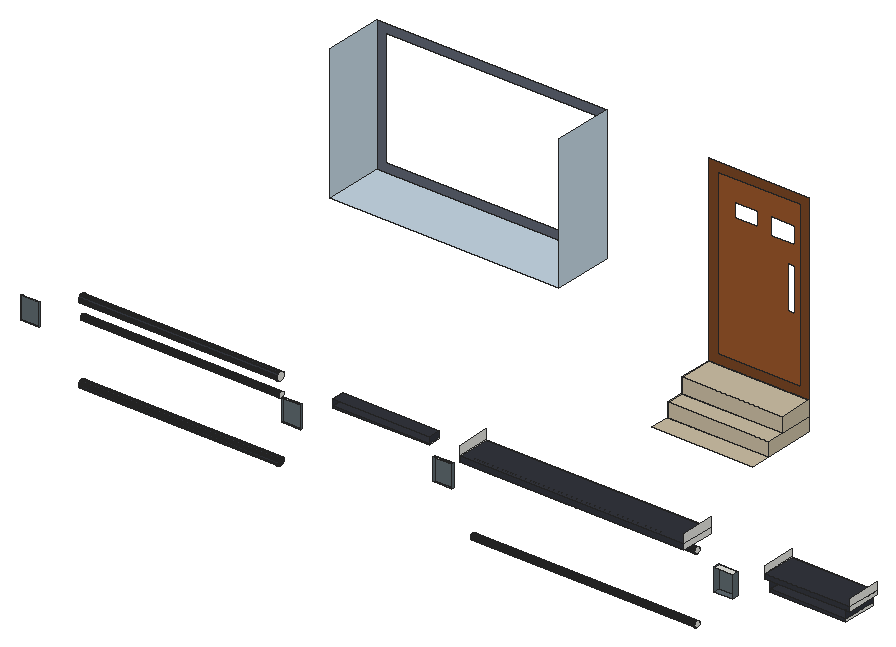
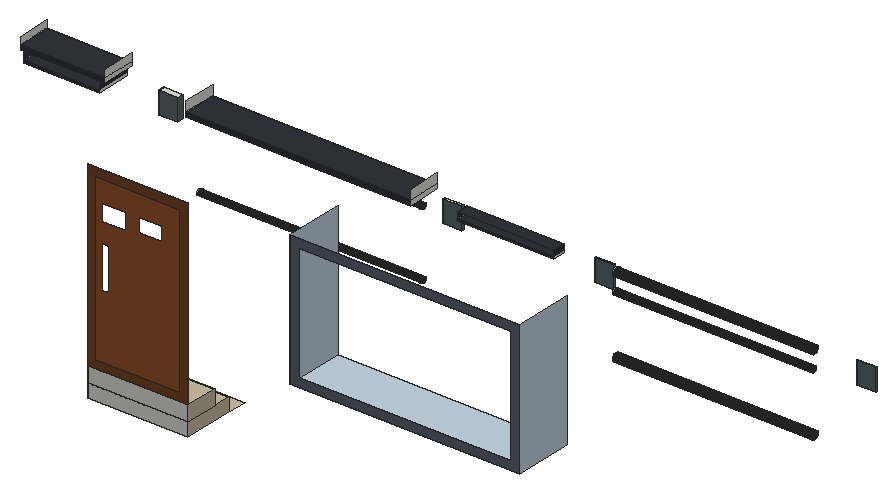
# SketchUp Ruby script. Lengths in inches.
U = 1.inch
M = Sketchup.active_model
def pt(a) = Geom::Point3d.new(a.map { |v| v * U })
def face(e, loops, mat)
  f = e.add_face(loops[0].map { |a| pt(a) })
  loops[1..].each { |l| e.add_face(l.map { |a| pt(a) }).erase! }
  f.material = f.back_material = mat if mat
  f
end
# faces: each face lists its corners as indices into pts; further lists are holes
def faces(e, pts, list, mat = nil) = list.each { |f| face(e, (f[0].is_a?(Array) ? f : [f]).map { |l| l.map { |i| pts[i] } }, mat) }
# xy, xz, yz: faces in a plane at the given z, y or x. An outline is a flat list of corners, or four numbers for a rectangle; further outlines are holes
def ring(l) = l.size == 4 ? [[l[0], l[1]], [l[2], l[1]], [l[2], l[3]], [l[0], l[3]]] : l.each_slice(2).to_a
def flat(e, list, mat, &to3) = list.each { |f| face(e, (f[0].is_a?(Array) ? f : [f]).map { |l| ring(l).map { |u, v| to3.(u, v) } }, mat) }
def xy(e, z, list, mat = nil) = flat(e, list, mat) { |x, y| [x, y, z] }
def xz(e, y, list, mat = nil) = flat(e, list, mat) { |x, z| [x, y, z] }
def yz(e, x, list, mat = nil) = flat(e, list, mat) { |y, z| [x, y, z] }
def lines(e, pts, list) = list.each { |a, b| e.add_line(pt(pts[a]), pt(pts[b])) }
# prism: a flat outline (further loops are holes) pulled along v
def prism(e, loops, v, mat = nil)
  f = face(e, loops, mat); d = Geom::Vector3d.new(v.map { |x| x * U })
  f.pushpull(f.normal.samedirection?(d) ? d.length : -d.length)
end
def box(e, o, s, mat = nil) = prism(e, [[o, [o[0] + s[0], o[1], o[2]], [o[0] + s[0], o[1] + s[1], o[2]], [o[0], o[1] + s[1], o[2]]]], [0, 0, s[2]], mat)
def at(x, y, z, deg = 0) = Geom::Transformation.translation(pt([x, y, z])) * Geom::Transformation.rotation(ORIGIN, Z_AXIS, deg.degrees)
def axes(o, x, y, z) = Geom::Transformation.new([*x, 0, *y, 0, *z, 0, *pt(o).to_a, 1])
def part(name) = M.definitions.add(name)
# library, detail: a bought-in or finely detailed component or shape, given as its bounding box
def library(name, o, s) = part(name).tap { |d| box(d.entities, o, s) }
def detail(e, o, s) = box(e.add_group.entities, o, s)
def put(e, d, t, mat = nil) = e.add_instance(d, t).tap { |i| i.material = mat if mat }
def group(e, t, mat = nil) = e.add_group.tap { |g| g.transformation = t; g.material = mat if mat }.entities
root = M.entities
M.materials.add("[Concrete Tile]").color = [203, 190, 164]
M.materials.add("[Formica Laminate Dark]").color = [95, 101, 114]
M.materials.add("[Formica Laminate Dark]1").color = [50, 53, 60]
M.materials.add("[Formica Speckled Grey]").color = [94, 105, 111]
M.materials.add("[Terrazzo Light Blue]1").color = [196, 214, 227]
M.materials.add("[Wood Cherry Original]").color = [152, 86, 42]
M.materials.add("[Wood Veneer 01]").color = [120, 70, 37]
xy(root,62.21,[[1882.4375,1041.58,2273.5625,1239.01]])
xy(root,62.21,[[1882.4375,963.83,2273.5625,1041.58]],"[Concrete Tile]")
xy(root,115.41,[[1882.4375,1110.33,2273.5625,1239.01]])
xy(root,115.41,[[1882.4375,1041.58,2273.5625,1110.33]],"[Concrete Tile]")
xy(root,172.83,[[1882.4375,1110.33,2273.5625,1239.01]],"[Concrete Tile]")
xy(root,268.73,[[199.14,0,272.27,4.5625],[1214.39,0,1287.52,6.3125],[1802.64,0,1875.77,7.75],[2895.58,0,2968.71,23.6875]],"[Formica Speckled Grey]")
xy(root,341.4375,[[2044.37,55.58,2046.83,56.09,2049.07,57.22,2050.95,58.9,2052.32,61,2053.11,63.38,2053.25,65.89,2052.74,68.35,2051.61,70.6,2049.9375,72.47,2047.84,73.85,2045.45,74.64,2042.94,74.78,2040.48,74.27,2038.24,73.14,2036.36,71.46,2034.99,69.36,2034.2,66.98,2034.06,64.47,2034.57,62.01,2035.7,59.76,2037.37,57.89,2039.47,56.51,2041.86,55.72]])
xy(root,341.625,[[2752.12,55.58,2754.58,56.09,2756.82,57.22,2758.7,58.9,2760.07,61,2760.86,63.38,2761,65.89,2760.49,68.35,2759.36,70.6,2757.6875,72.47,2755.59,73.85,2753.2,74.64,2750.69,74.78,2748.23,74.27,2745.99,73.14,2744.11,71.46,2742.74,69.36,2741.95,66.98,2741.81,64.47,2742.32,62.01,2743.45,59.76,2745.12,57.89,2747.22,56.51,2749.61,55.72]])
xy(root,342.54,[[[3111.49,0,3407.39,129.42],[3376.3,55.58,3378.76,56.09,3381.01,57.22,3382.88,58.9,3384.26,61,3385.05,63.38,3385.19,65.89,3384.68,68.35,3383.55,70.6,3381.875,72.47,3379.77,73.85,3377.39,74.64,3374.88,74.78,3372.42,74.27,3370.18,73.14,3368.3,71.46,3366.92,69.36,3366.14,66.98,3365.99,64.47,3366.51,62.01,3367.64,59.76,3369.31,57.89,3371.41,56.51,3373.8,55.72],[3328.68,55.58,3331.14,56.09,3333.38,57.22,3335.26,58.9,3336.64,61,3337.42,63.38,3337.57,65.89,3337.05,68.35,3335.92,70.6,3334.25,72.47,3332.15,73.85,3329.76,74.64,3327.25,74.78,3324.79,74.27,3322.55,73.14,3320.68,71.46,3319.3,69.36,3318.51,66.98,3318.37,64.47,3318.88,62.01,3320.01,59.76,3321.68,57.89,3323.79,56.51,3326.17,55.72],[3282.55,55.58,3285.01,56.09,3287.26,57.22,3289.13,58.9,3290.51,61,3291.3,63.38,3291.44,65.89,3290.93,68.35,3289.8,70.6,3288.125,72.47,3286.02,73.85,3283.64,74.64,3281.13,74.78,3278.67,74.27,3276.43,73.14,3274.55,71.46,3273.17,69.36,3272.39,66.98,3272.24,64.47,3272.76,62.01,3273.89,59.76,3275.56,57.89,3277.66,56.51,3280.05,55.72],[3236.93,55.58,3239.39,56.09,3241.63,57.22,3243.51,58.9,3244.89,61,3245.67,63.38,3245.82,65.89,3245.3,68.35,3244.17,70.6,3242.5,72.47,3240.4,73.85,3238.01,74.64,3235.5,74.78,3233.04,74.27,3230.8,73.14,3228.93,71.46,3227.55,69.36,3226.76,66.98,3226.62,64.47,3227.13,62.01,3228.26,59.76,3229.93,57.89,3232.04,56.51,3234.42,55.72],[3187.99,55.58,3190.45,56.09,3192.7,57.22,3194.57,58.9,3195.95,61,3196.74,63.38,3196.88,65.89,3196.37,68.35,3195.24,70.6,3193.5625,72.47,3191.46,73.85,3189.08,74.64,3186.57,74.78,3184.11,74.27,3181.86,73.14,3179.99,71.46,3178.61,69.36,3177.82,66.98,3177.68,64.47,3178.19,62.01,3179.32,59.76,3181,57.89,3183.1,56.51,3185.48,55.72],[3137.87,55.58,3140.33,56.09,3142.57,57.22,3144.45,58.9,3145.82,61,3146.61,63.38,3146.75,65.89,3146.24,68.35,3145.11,70.6,3143.4375,72.47,3141.34,73.85,3138.95,74.64,3136.44,74.78,3133.98,74.27,3131.74,73.14,3129.86,71.46,3128.49,69.36,3127.7,66.98,3127.56,64.47,3128.07,62.01,3129.2,59.76,3130.87,57.89,3132.97,56.51,3135.36,55.72]]],"[Formica Laminate Dark]1")
xy(root,342.8,[[2139.99,55.58,2142.45,56.09,2144.7,57.22,2146.57,58.9,2147.95,61,2148.74,63.38,2148.88,65.89,2148.37,68.35,2147.24,70.6,2145.5625,72.47,2143.46,73.85,2141.08,74.64,2138.57,74.78,2136.11,74.27,2133.86,73.14,2131.99,71.46,2130.61,69.36,2129.82,66.98,2129.68,64.47,2130.19,62.01,2131.32,59.76,2133,57.89,2135.1,56.51,2137.48,55.72],[2458.12,55.58,2460.58,56.09,2462.82,57.22,2464.7,58.9,2466.07,61,2466.86,63.38,2467,65.89,2466.49,68.35,2465.36,70.6,2463.6875,72.47,2461.59,73.85,2459.2,74.64,2456.69,74.78,2454.23,74.27,2451.99,73.14,2450.11,71.46,2448.74,69.36,2447.95,66.98,2447.81,64.47,2448.32,62.01,2449.45,59.76,2451.12,57.89,2453.22,56.51,2455.61,55.72],[2700.93,55.58,2703.39,56.09,2705.63,57.22,2707.51,58.9,2708.89,61,2709.67,63.38,2709.82,65.89,2709.3,68.35,2708.17,70.6,2706.5,72.47,2704.4,73.85,2702.01,74.64,2699.5,74.78,2697.04,74.27,2694.8,73.14,2692.93,71.46,2691.55,69.36,2690.76,66.98,2690.62,64.47,2691.13,62.01,2692.26,59.76,2693.93,57.89,2696.04,56.51,2698.42,55.72]])
xy(root,343.0625,[[2187.99,55.58,2190.45,56.09,2192.7,57.22,2194.57,58.9,2195.95,61,2196.74,63.38,2196.88,65.89,2196.37,68.35,2195.24,70.6,2193.5625,72.47,2191.46,73.85,2189.08,74.64,2186.57,74.78,2184.11,74.27,2181.86,73.14,2179.99,71.46,2178.61,69.36,2177.82,66.98,2177.68,64.47,2178.19,62.01,2179.32,59.76,2181,57.89,2183.1,56.51,2185.48,55.72]])
xy(root,343.5,[[1934.18,55.58,1936.64,56.09,1938.88,57.22,1940.76,58.9,1942.14,61,1942.92,63.38,1943.07,65.89,1942.55,68.35,1941.42,70.6,1939.75,72.47,1937.65,73.85,1935.26,74.64,1932.75,74.78,1930.29,74.27,1928.05,73.14,1926.18,71.46,1924.8,69.36,1924.01,66.98,1923.87,64.47,1924.38,62.01,1925.51,59.76,1927.18,57.89,1929.29,56.51,1931.67,55.72]])
xy(root,343.625,[[2404.12,55.58,2406.58,56.09,2408.82,57.22,2410.7,58.9,2412.07,61,2412.86,63.38,2413,65.89,2412.49,68.35,2411.36,70.6,2409.6875,72.47,2407.59,73.85,2405.2,74.64,2402.69,74.78,2400.23,74.27,2397.99,73.14,2396.11,71.46,2394.74,69.36,2393.95,66.98,2393.81,64.47,2394.32,62.01,2395.45,59.76,2397.12,57.89,2399.22,56.51,2401.61,55.72]])
xy(root,344.25,[[2557.49,55.58,2559.95,56.09,2562.2,57.22,2564.07,58.9,2565.45,61,2566.24,63.38,2566.38,65.89,2565.87,68.35,2564.74,70.6,2563.0625,72.47,2560.96,73.85,2558.58,74.64,2556.07,74.78,2553.61,74.27,2551.36,73.14,2549.49,71.46,2548.11,69.36,2547.32,66.98,2547.18,64.47,2547.69,62.01,2548.82,59.76,2550.5,57.89,2552.6,56.51,2554.98,55.72]])
xy(root,344.375,[[2604.55,55.58,2607.01,56.09,2609.26,57.22,2611.13,58.9,2612.51,61,2613.3,63.38,2613.44,65.89,2612.93,68.35,2611.8,70.6,2610.125,72.47,2608.02,73.85,2605.64,74.64,2603.13,74.78,2600.67,74.27,2598.43,73.14,2596.55,71.46,2595.17,69.36,2594.39,66.98,2594.24,64.47,2594.76,62.01,2595.89,59.76,2597.56,57.89,2599.66,56.51,2602.05,55.72]])
xy(root,345,[[2508.93,55.58,2511.39,56.09,2513.63,57.22,2515.51,58.9,2516.89,61,2517.67,63.38,2517.82,65.89,2517.3,68.35,2516.17,70.6,2514.5,72.47,2512.4,73.85,2510.01,74.64,2507.5,74.78,2505.04,74.27,2502.8,73.14,2500.93,71.46,2499.55,69.36,2498.76,66.98,2498.62,64.47,2499.13,62.01,2500.26,59.76,2501.93,57.89,2504.04,56.51,2506.42,55.72]])
xy(root,345.54,[[1991.49,55.58,1993.95,56.09,1996.2,57.22,1998.07,58.9,1999.45,61,2000.24,63.38,2000.38,65.89,1999.87,68.35,1998.74,70.6,1997.0625,72.47,1994.96,73.85,1992.58,74.64,1990.07,74.78,1987.61,74.27,1985.36,73.14,1983.49,71.46,1982.11,69.36,1981.32,66.98,1981.18,64.47,1981.69,62.01,1982.82,59.76,1984.5,57.89,1986.6,56.51,1988.98,55.72]])
xy(root,346,[[2651.93,55.58,2654.39,56.09,2656.63,57.22,2658.51,58.9,2659.89,61,2660.67,63.38,2660.82,65.89,2660.3,68.35,2659.17,70.6,2657.5,72.47,2655.4,73.85,2653.01,74.64,2650.5,74.78,2648.04,74.27,2645.8,73.14,2643.93,71.46,2642.55,69.36,2641.76,66.98,2641.62,64.47,2642.13,62.01,2643.26,59.76,2644.93,57.89,2647.04,56.51,2649.42,55.72]])
xy(root,346.125,[[2286.99,55.58,2289.45,56.09,2291.7,57.22,2293.57,58.9,2294.95,61,2295.74,63.38,2295.88,65.89,2295.37,68.35,2294.24,70.6,2292.5625,72.47,2290.46,73.85,2288.08,74.64,2285.57,74.78,2283.11,74.27,2280.86,73.14,2278.99,71.46,2277.61,69.36,2276.82,66.98,2276.68,64.47,2277.19,62.01,2278.32,59.76,2280,57.89,2282.1,56.51,2284.48,55.72]])
xy(root,347.25,[[2094.55,55.58,2097.01,56.09,2099.26,57.22,2101.13,58.9,2102.51,61,2103.3,63.38,2103.44,65.89,2102.93,68.35,2101.8,70.6,2100.125,72.47,2098.02,73.85,2095.64,74.64,2093.13,74.78,2090.67,74.27,2088.43,73.14,2086.55,71.46,2085.17,69.36,2084.39,66.98,2084.24,64.47,2084.76,62.01,2085.89,59.76,2087.56,57.89,2089.66,56.51,2092.05,55.72]])
xy(root,347.3125,[[2238.68,55.58,2241.14,56.09,2243.38,57.22,2245.26,58.9,2246.64,61,2247.42,63.38,2247.57,65.89,2247.05,68.35,2245.92,70.6,2244.25,72.47,2242.15,73.85,2239.76,74.64,2237.25,74.78,2234.79,74.27,2232.55,73.14,2230.68,71.46,2229.3,69.36,2228.51,66.98,2228.37,64.47,2228.88,62.01,2230.01,59.76,2231.68,57.89,2233.79,56.51,2236.17,55.72]])
xy(root,353.375,[[3111.49,0,3407.39,129.42]],"[Formica Laminate Dark]1")
xy(root,354.42,[[199.14,0,272.27,4.5625],[1214.39,0,1287.52,6.3125],[1802.64,0,1875.77,7.75],[2895.58,0,2968.71,23.6875]])
xy(root,357.02,[[[1376.86,44.85,1752.89,92.78],[1417.24,55.58,1419.7,56.09,1421.95,57.22,1423.82,58.9,1425.2,61,1425.99,63.38,1426.13,65.89,1425.62,68.35,1424.49,70.6,1422.8125,72.47,1420.71,73.85,1418.33,74.64,1415.82,74.78,1413.36,74.27,1411.11,73.14,1409.24,71.46,1407.86,69.36,1407.07,66.98,1406.93,64.47,1407.44,62.01,1408.57,59.76,1410.25,57.89,1412.35,56.51,1414.73,55.72],[1472.87,55.58,1475.33,56.09,1477.57,57.22,1479.45,58.9,1480.82,61,1481.61,63.38,1481.75,65.89,1481.24,68.35,1480.11,70.6,1478.4375,72.47,1476.34,73.85,1473.95,74.64,1471.44,74.78,1468.98,74.27,1466.74,73.14,1464.86,71.46,1463.49,69.36,1462.7,66.98,1462.56,64.47,1463.07,62.01,1464.2,59.76,1465.87,57.89,1467.97,56.51,1470.36,55.72],[1518.99,55.58,1521.45,56.09,1523.7,57.22,1525.57,58.9,1526.95,61,1527.74,63.38,1527.88,65.89,1527.37,68.35,1526.24,70.6,1524.5625,72.47,1522.46,73.85,1520.08,74.64,1517.57,74.78,1515.11,74.27,1512.86,73.14,1510.99,71.46,1509.61,69.36,1508.82,66.98,1508.68,64.47,1509.19,62.01,1510.32,59.76,1512,57.89,1514.1,56.51,1516.48,55.72],[1566.87,55.58,1569.33,56.09,1571.57,57.22,1573.45,58.9,1574.82,61,1575.61,63.38,1575.75,65.89,1575.24,68.35,1574.11,70.6,1572.4375,72.47,1570.34,73.85,1567.95,74.64,1565.44,74.78,1562.98,74.27,1560.74,73.14,1558.86,71.46,1557.49,69.36,1556.7,66.98,1556.56,64.47,1557.07,62.01,1558.2,59.76,1559.87,57.89,1561.97,56.51,1564.36,55.72],[1616.43,55.58,1618.89,56.09,1621.13,57.22,1623.01,58.9,1624.39,61,1625.17,63.38,1625.32,65.89,1624.8,68.35,1623.67,70.6,1622,72.47,1619.9,73.85,1617.51,74.64,1615,74.78,1612.54,74.27,1610.3,73.14,1608.43,71.46,1607.05,69.36,1606.26,66.98,1606.12,64.47,1606.63,62.01,1607.76,59.76,1609.43,57.89,1611.54,56.51,1613.92,55.72],[1663.87,55.58,1666.33,56.09,1668.57,57.22,1670.45,58.9,1671.82,61,1672.61,63.38,1672.75,65.89,1672.24,68.35,1671.11,70.6,1669.4375,72.47,1667.34,73.85,1664.95,74.64,1662.44,74.78,1659.98,74.27,1657.74,73.14,1655.86,71.46,1654.49,69.36,1653.7,66.98,1653.56,64.47,1654.07,62.01,1655.2,59.76,1656.87,57.89,1658.97,56.51,1661.36,55.72],[1714.37,55.58,1716.83,56.09,1719.07,57.22,1720.95,58.9,1722.32,61,1723.11,63.38,1723.25,65.89,1722.74,68.35,1721.61,70.6,1719.9375,72.47,1717.84,73.85,1715.45,74.64,1712.94,74.78,1710.48,74.27,1708.24,73.14,1706.36,71.46,1704.99,69.36,1704.2,66.98,1704.06,64.47,1704.57,62.01,1705.7,59.76,1707.37,57.89,1709.47,56.51,1711.86,55.72]]],"[Formica Laminate Dark]1")
xy(root,362.53,[[1376.86,44.85,1752.89,92.78]],"[Formica Laminate Dark]1")
xy(root,373.4375,[[465.05,55.58,467.51,56.09,469.76,57.22,471.63,58.9,473.01,61,473.8,63.38,473.94,65.89,473.43,68.35,472.3,70.6,470.625,72.47,468.52,73.85,466.14,74.64,463.63,74.78,461.17,74.27,458.93,73.14,457.05,71.46,455.67,69.36,454.89,66.98,454.74,64.47,455.26,62.01,456.39,59.76,458.06,57.89,460.16,56.51,462.55,55.72]])
xy(root,373.47,[[2358.7,0,2386.55,129.42]])
xy(root,373.47,[[1905.75,0,2330.84,129.42],[2386.55,0,2778.47,129.42]],"[Formica Laminate Dark]1")
xy(root,374.5625,[[648.8,55.58,651.26,56.09,653.51,57.22,655.38,58.9,656.76,61,657.55,63.38,657.69,65.89,657.18,68.35,656.05,70.6,654.375,72.47,652.27,73.85,649.89,74.64,647.38,74.78,644.92,74.27,642.68,73.14,640.8,71.46,639.42,69.36,638.64,66.98,638.49,64.47,639.01,62.01,640.14,59.76,641.81,57.89,643.91,56.51,646.3,55.72]])
xy(root,374.6875,[[525.12,55.58,527.58,56.09,529.82,57.22,531.7,58.9,533.07,61,533.86,63.38,534,65.89,533.49,68.35,532.36,70.6,530.6875,72.47,528.59,73.85,526.2,74.64,523.69,74.78,521.23,74.27,518.99,73.14,517.11,71.46,515.74,69.36,514.95,66.98,514.81,64.47,515.32,62.01,516.45,59.76,518.12,57.89,520.22,56.51,522.61,55.72]])
xy(root,375.0625,[[1102.12,55.58,1104.58,56.09,1106.82,57.22,1108.7,58.9,1110.07,61,1110.86,63.38,1111,65.89,1110.49,68.35,1109.36,70.6,1107.6875,72.47,1105.59,73.85,1103.2,74.64,1100.69,74.78,1098.23,74.27,1095.99,73.14,1094.11,71.46,1092.74,69.36,1091.95,66.98,1091.81,64.47,1092.32,62.01,1093.45,59.76,1095.12,57.89,1097.22,56.51,1099.61,55.72]])
xy(root,376.5,[[777.12,55.58,779.58,56.09,781.82,57.22,783.7,58.9,785.07,61,785.86,63.38,786,65.89,785.49,68.35,784.36,70.6,782.6875,72.47,780.59,73.85,778.2,74.64,775.69,74.78,773.23,74.27,770.99,73.14,769.11,71.46,767.74,69.36,766.95,66.98,766.81,64.47,767.32,62.01,768.45,59.76,770.12,57.89,772.22,56.51,774.61,55.72]])
xy(root,378.25,[[714.12,55.58,716.58,56.09,718.82,57.22,720.7,58.9,722.07,61,722.86,63.38,723,65.89,722.49,68.35,721.36,70.6,719.6875,72.47,717.59,73.85,715.2,74.64,712.69,74.78,710.23,74.27,707.99,73.14,706.11,71.46,704.74,69.36,703.95,66.98,703.81,64.47,704.32,62.01,705.45,59.76,707.12,57.89,709.22,56.51,711.61,55.72]])
xy(root,378.85,[[585.24,55.58,587.7,56.09,589.95,57.22,591.82,58.9,593.2,61,593.99,63.38,594.13,65.89,593.62,68.35,592.49,70.6,590.8125,72.47,588.71,73.85,586.33,74.64,583.82,74.78,581.36,74.27,579.11,73.14,577.24,71.46,575.86,69.36,575.07,66.98,574.93,64.47,575.44,62.01,576.57,59.76,578.25,57.89,580.35,56.51,582.73,55.72],[840.24,55.58,842.7,56.09,844.95,57.22,846.82,58.9,848.2,61,848.99,63.38,849.13,65.89,848.62,68.35,847.49,70.6,845.8125,72.47,843.71,73.85,841.33,74.64,838.82,74.78,836.36,74.27,834.11,73.14,832.24,71.46,830.86,69.36,830.07,66.98,829.93,64.47,830.44,62.01,831.57,59.76,833.25,57.89,835.35,56.51,837.73,55.72]])
xy(root,379.125,[[905.18,55.58,907.64,56.09,909.88,57.22,911.76,58.9,913.14,61,913.92,63.38,914.07,65.89,913.55,68.35,912.42,70.6,910.75,72.47,908.65,73.85,906.26,74.64,903.75,74.78,901.29,74.27,899.05,73.14,897.18,71.46,895.8,69.36,895.01,66.98,894.87,64.47,895.38,62.01,896.51,59.76,898.18,57.89,900.29,56.51,902.67,55.72]])
xy(root,381.875,[[1034.62,55.58,1037.08,56.09,1039.32,57.22,1041.2,58.9,1042.57,61,1043.36,63.38,1043.5,65.89,1042.99,68.35,1041.86,70.6,1040.1875,72.47,1038.09,73.85,1035.7,74.64,1033.19,74.78,1030.73,74.27,1028.49,73.14,1026.61,71.46,1025.24,69.36,1024.45,66.98,1024.31,64.47,1024.82,62.01,1025.95,59.76,1027.62,57.89,1029.72,56.51,1032.11,55.72]])
xy(root,384.04,[[3092.67,0,3111.49,129.42],[3407.39,0,3421.78,129.42]])
xy(root,384.04,[[3111.49,0,3407.39,129.42]],"[Formica Laminate Dark]1")
xy(root,384.0625,[[968.99,55.58,971.45,56.09,973.7,57.22,975.57,58.9,976.95,61,977.74,63.38,977.88,65.89,977.37,68.35,976.24,70.6,974.5625,72.47,972.46,73.85,970.08,74.64,967.57,74.78,965.11,74.27,962.86,73.14,960.99,71.46,959.61,69.36,958.82,66.98,958.68,64.47,959.19,62.01,960.32,59.76,962,57.89,964.1,56.51,966.48,55.72]])
xy(root,386.38,[[416.3,55.58,418.76,56.09,421.01,57.22,422.88,58.9,424.26,61,425.05,63.38,425.19,65.89,424.68,68.35,423.55,70.6,421.875,72.47,419.77,73.85,417.39,74.64,414.88,74.78,412.42,74.27,410.18,73.14,408.3,71.46,406.92,69.36,406.14,66.98,405.99,64.47,406.51,62.01,407.64,59.76,409.31,57.89,411.41,56.51,413.8,55.72]])
xy(root,387.41,[[594.7,1008.89,1485.01,1239.01]],"[Terrazzo Light Blue]1")
xy(root,387.92,[[1376.86,44.85,1752.89,92.78]],"[Formica Laminate Dark]1")
xy(root,392.18,[[1905.75,0,2778.47,129.42]],"[Formica Laminate Dark]1")
xy(root,400.8,[[3092.67,0,3421.78,129.42]],"[Formica Laminate Dark]1")
xz(root,0,[[3111.49,342.54,3407.39,353.375],[1905.75,373.47,2778.47,392.18],[3092.67,384.04,3421.78,400.8]],"[Formica Laminate Dark]1")
xz(root,4.5625,[[199.14,268.73,272.27,354.42]],"[Formica Speckled Grey]")
xz(root,6.3125,[[1214.39,268.73,1287.52,354.42]],"[Formica Speckled Grey]")
xz(root,7.75,[[1802.64,268.73,1875.77,354.42]],"[Formica Speckled Grey]")
xz(root,23.6875,[[2895.58,268.73,2968.71,354.42]],"[Formica Speckled Grey]")
xz(root,44.85,[[1376.86,357.02,1752.89,362.53]],"[Formica Laminate Dark]1")
xz(root,92.78,[[1376.86,357.02,1752.89,362.53]],"[Formica Laminate Dark]1")
xz(root,129.42,[[3111.49,342.54,3407.39,353.375],[1905.75,373.47,2778.47,392.18],[3092.67,384.04,3421.78,400.8]],"[Formica Laminate Dark]1")
xz(root,1041.58,[[1882.4375,62.21,2273.5625,115.41]],"[Concrete Tile]")
xz(root,1110.33,[[1882.4375,115.41,2273.5625,172.83]],"[Concrete Tile]")
xz(root,1239.01,[[1882.4375,62.21,2273.5625,115.41],[1882.4375,115.41,2273.5625,172.83]])
xz(root,1239.01,[[[594.7,387.41,1485.01,905.79],[627.24,419.96,1452.47,873.24]]],"[Formica Laminate Dark]")
xz(root,1239.01,[[[1916.82,207.21,2239.18,842.83],[2125.16,693.23,2217.66,761.05],[1985.88,705.68,2074.875,760.68],[2190.67,454.58,2217.05,620.33]]],"[Wood Cherry Original]")
xz(root,1239.01,[[[1882.4375,172.83,2273.5625,877.21],[1916.82,207.21,2239.18,842.83]]],"[Wood Veneer 01]")
yz(root,199.14,[[0,268.73,4.5625,354.42]],"[Formica Speckled Grey]")
yz(root,272.27,[[0,268.73,4.5625,354.42]],"[Formica Speckled Grey]")
yz(root,594.7,[[1008.89,387.41,1239.01,905.79]],"[Terrazzo Light Blue]1")
yz(root,1157.35,[[71.79,301.92,74.46,302.27,76.94,303.3,79.08,304.9375,80.72,307.07,81.75,309.5625,82.1,312.23,81.75,314.9,80.72,317.39,79.08,319.52,76.94,321.16,74.46,322.19,71.79,322.54,69.12,322.19,66.63,321.16,64.5,319.52,62.86,317.39,61.83,314.9,61.48,312.23,61.83,309.5625,62.86,307.07,64.5,304.9375,66.63,303.3,69.12,302.27],[67.74,363.79,71.64,364.3,75.27,365.81,78.39,368.2,80.79,371.32,82.29,374.95,82.81,378.85,82.29,382.75,80.79,386.38,78.39,389.5,75.27,391.9,71.64,393.4,67.74,393.92,63.84,393.4,60.21,391.9,57.09,389.5,54.7,386.38,53.19,382.75,52.68,378.85,53.19,374.95,54.7,371.32,57.09,368.2,60.21,365.81,63.84,364.3]])
yz(root,1214.39,[[0,268.73,6.3125,354.42]],"[Formica Speckled Grey]")
yz(root,1287.52,[[0,268.73,6.3125,354.42]],"[Formica Speckled Grey]")
yz(root,1376.86,[[44.85,357.02,92.78,362.53]])
yz(root,1376.86,[[44.85,362.53,92.78,387.92]],"[Formica Laminate Dark]1")
yz(root,1485.01,[[1008.89,387.41,1239.01,905.79]],"[Terrazzo Light Blue]1")
yz(root,1752.89,[[44.85,357.02,92.78,362.53]])
yz(root,1752.89,[[44.85,362.53,92.78,387.92]],"[Formica Laminate Dark]1")
yz(root,1802.64,[[0,268.73,7.75,354.42]],"[Formica Speckled Grey]")
yz(root,1875.77,[[0,268.73,7.75,354.42]],"[Formica Speckled Grey]")
yz(root,1882.4375,[[1041.58,62.21,1239.01,115.41],[1110.33,115.41,1239.01,172.83]],"[Concrete Tile]")
yz(root,1905.75,[[0,373.47,129.42,392.18],[0,392.18,129.42,429.3125]])
yz(root,2273.5625,[[1041.58,62.21,1239.01,115.41],[1110.33,115.41,1239.01,172.83]],"[Concrete Tile]")
yz(root,2778.47,[[64.71,75.12,67.44,75.48,69.99,76.53,72.18,78.21,73.86,80.4,74.91,82.94,75.27,85.68,74.91,88.41,73.86,90.96,72.18,93.15,69.99,94.83,67.44,95.88,64.71,96.24,61.98,95.88,59.43,94.83,57.24,93.15,55.5625,90.96,54.51,88.41,54.15,85.68,54.51,82.94,55.5625,80.4,57.24,78.21,59.43,76.53,61.98,75.48],[64.71,332.24,67.44,332.6,69.99,333.66,72.18,335.33,73.86,337.52,74.91,340.07,75.27,342.8,74.91,345.54,73.86,348.08,72.18,350.27,69.99,351.95,67.44,353.01,64.71,353.37,61.98,353.01,59.43,351.95,57.24,350.27,55.5625,348.08,54.51,345.54,54.15,342.8,54.51,340.07,55.5625,337.52,57.24,335.33,59.43,333.66,61.98,332.6],[0,373.47,129.42,392.18],[0,392.18,129.42,429.3125]])
yz(root,2895.58,[[0,268.73,23.6875,354.42]],"[Formica Speckled Grey]")
yz(root,2968.71,[[0,268.73,23.6875,354.42]],"[Formica Speckled Grey]")
yz(root,3092.67,[[0,384.04,129.42,400.8],[0,400.8,129.42,429.3125]])
yz(root,3111.49,[[0,342.54,129.42,353.375]])
yz(root,3111.49,[[0,353.375,129.42,384.04]],"[Formica Laminate Dark]1")
yz(root,3407.39,[[0,342.54,129.42,353.375]])
yz(root,3407.39,[[0,353.375,129.42,384.04]],"[Formica Laminate Dark]1")
yz(root,3421.78,[[0,384.04,129.42,400.8],[0,400.8,129.42,429.3125]])
p = [[1157.35,67.74,66.35],[1157.35,63.84,66.87],[383.65,63.84,66.87],[383.65,67.74,66.35],[1157.35,71.64,66.87],[383.65,71.64,66.87],
  [1157.35,60.21,68.37],[383.65,60.21,68.37],[1157.35,75.27,68.37],[383.65,75.27,68.37],[1157.35,57.09,70.76],[383.65,57.09,70.76],
  [1157.35,78.39,70.76],[383.65,78.39,70.76],[1157.35,54.7,73.88],[383.65,54.7,73.88],[1157.35,80.79,73.88],[383.65,80.79,73.88],
  [1157.35,53.19,77.52],[383.65,53.19,77.52],[1157.35,82.29,77.52],[383.65,82.29,77.52],[2778.47,64.71,75.12],[2778.47,61.98,75.48],
  [1905.75,61.98,75.48],[1905.75,64.71,75.12],[2778.47,67.44,75.48],[1905.75,67.44,75.48],[2778.47,59.43,76.53],[1905.75,59.43,76.53],
  [2778.47,69.99,76.53],[1905.75,69.99,76.53],[2778.47,57.24,78.21],[1905.75,57.24,78.21],[2778.47,72.18,78.21],[1905.75,72.18,78.21],
  [1157.35,52.68,81.42],[383.65,52.68,81.42],[1157.35,82.81,81.42],[383.65,82.81,81.42],[2778.47,55.5625,80.4],[1905.75,55.5625,80.4],
  [2778.47,73.86,80.4],[1905.75,73.86,80.4],[2778.47,54.51,82.94],[1905.75,54.51,82.94],[2778.47,74.91,82.94],[1905.75,74.91,82.94],
  [1157.35,53.19,85.3125],[383.65,53.19,85.3125],[1157.35,82.29,85.3125],[383.65,82.29,85.3125],[2778.47,54.15,85.68],[1905.75,54.15,85.68],
  [2778.47,75.27,85.68],[1905.75,75.27,85.68],[1157.35,54.7,88.95],[383.65,54.7,88.95],[1157.35,80.79,88.95],[383.65,80.79,88.95],
  [2778.47,54.51,88.41],[1905.75,54.51,88.41],[2778.47,74.91,88.41],[1905.75,74.91,88.41],[2778.47,55.5625,90.96],[1905.75,55.5625,90.96],
  [2778.47,73.86,90.96],[1905.75,73.86,90.96],[1157.35,57.09,92.07],[383.65,57.09,92.07],[1157.35,78.39,92.07],[383.65,78.39,92.07],
  [2778.47,57.24,93.15],[1905.75,57.24,93.15],[2778.47,72.18,93.15],[1905.75,72.18,93.15],[1157.35,60.21,94.46],[383.65,60.21,94.46],
  [1157.35,75.27,94.46],[383.65,75.27,94.46],[2778.47,59.43,94.83],[1905.75,59.43,94.83],[2778.47,69.99,94.83],[1905.75,69.99,94.83],
  [1157.35,63.84,95.96],[383.65,63.84,95.96],[1157.35,71.64,95.96],[383.65,71.64,95.96],[2778.47,61.98,95.88],[1905.75,61.98,95.88],
  [2778.47,67.44,95.88],[1905.75,67.44,95.88],[2778.47,64.71,96.24],[1905.75,64.71,96.24],[1157.35,67.74,96.48],[383.65,67.74,96.48],
  [1157.35,71.79,301.92],[1157.35,69.12,302.27],[383.65,69.12,302.27],[383.65,71.79,301.92],[1157.35,74.46,302.27],[383.65,74.46,302.27],
  [1157.35,66.63,303.3],[383.65,66.63,303.3],[1157.35,76.94,303.3],[383.65,76.94,303.3],[1157.35,64.5,304.9375],[383.65,64.5,304.9375],
  [1157.35,79.08,304.9375],[383.65,79.08,304.9375],[1157.35,62.86,307.07],[383.65,62.86,307.07],[1157.35,80.72,307.07],[383.65,80.72,307.07],
  [1157.35,61.83,309.5625],[383.65,61.83,309.5625],[1157.35,81.75,309.5625],[383.65,81.75,309.5625],[1157.35,61.48,312.23],[383.65,61.48,312.23],
  [1157.35,82.1,312.23],[383.65,82.1,312.23],[1157.35,61.83,314.9],[383.65,61.83,314.9],[1157.35,81.75,314.9],[383.65,81.75,314.9],
  [1157.35,62.86,317.39],[383.65,62.86,317.39],[1157.35,80.72,317.39],[383.65,80.72,317.39],[1157.35,64.5,319.52],[383.65,64.5,319.52],
  [1157.35,79.08,319.52],[383.65,79.08,319.52],[1157.35,66.63,321.16],[383.65,66.63,321.16],[1157.35,76.94,321.16],[383.65,76.94,321.16],
  [1157.35,69.12,322.19],[383.65,69.12,322.19],[1157.35,74.46,322.19],[383.65,74.46,322.19],[1157.35,71.79,322.54],[383.65,71.79,322.54],
  [2778.47,64.71,332.24],[2778.47,61.98,332.6],[1905.75,61.98,332.6],[1905.75,64.71,332.24],[2778.47,67.44,332.6],[1905.75,67.44,332.6],
  [2778.47,59.43,333.66],[1905.75,59.43,333.66],[2778.47,69.99,333.66],[1905.75,69.99,333.66],[2778.47,57.24,335.33],[1905.75,57.24,335.33],
  [2778.47,72.18,335.33],[1905.75,72.18,335.33],[2778.47,55.5625,337.52],[1905.75,55.5625,337.52],[2778.47,73.86,337.52],[1905.75,73.86,337.52],
  [2778.47,54.51,340.07],[1905.75,54.51,340.07],[2778.47,74.91,340.07],[1905.75,74.91,340.07],[2778.47,54.15,342.8],[1905.75,54.15,342.8],
  [2778.47,75.27,342.8],[1905.75,75.27,342.8],[2778.47,54.51,345.54],[1905.75,54.51,345.54],[2778.47,74.91,345.54],[1905.75,74.91,345.54],
  [2778.47,55.5625,348.08],[1905.75,55.5625,348.08],[2778.47,73.86,348.08],[1905.75,73.86,348.08],[2778.47,57.24,350.27],[1905.75,57.24,350.27],
  [2778.47,72.18,350.27],[1905.75,72.18,350.27],[2778.47,59.43,351.95],[1905.75,59.43,351.95],[2778.47,69.99,351.95],[1905.75,69.99,351.95],
  [2778.47,61.98,353.01],[1905.75,61.98,353.01],[2778.47,67.44,353.01],[1905.75,67.44,353.01],[2778.47,64.71,353.37],[1905.75,64.71,353.37],
  [1157.35,67.74,363.79],[1157.35,63.84,364.3],[383.65,63.84,364.3],[383.65,67.74,363.79],[1157.35,71.64,364.3],[383.65,71.64,364.3],
  [1157.35,60.21,365.81],[383.65,60.21,365.81],[1157.35,75.27,365.81],[383.65,75.27,365.81],[1157.35,57.09,368.2],[383.65,57.09,368.2],
  [1157.35,78.39,368.2],[383.65,78.39,368.2],[1157.35,54.7,371.32],[383.65,54.7,371.32],[1157.35,80.79,371.32],[383.65,80.79,371.32],
  [1157.35,53.19,374.95],[383.65,53.19,374.95],[1157.35,82.29,374.95],[383.65,82.29,374.95],[1157.35,52.68,378.85],[383.65,52.68,378.85],
  [1157.35,82.81,378.85],[383.65,82.81,378.85],[1157.35,53.19,382.75],[383.65,53.19,382.75],[1157.35,82.29,382.75],[383.65,82.29,382.75],
  [1157.35,54.7,386.38],[383.65,54.7,386.38],[1157.35,80.79,386.38],[383.65,80.79,386.38],[1157.35,57.09,389.5],[383.65,57.09,389.5],
  [1157.35,78.39,389.5],[383.65,78.39,389.5],[1157.35,60.21,391.9],[383.65,60.21,391.9],[1157.35,75.27,391.9],[383.65,75.27,391.9],
  [1157.35,63.84,393.4],[383.65,63.84,393.4],[1157.35,71.64,393.4],[383.65,71.64,393.4],[1157.35,67.74,393.92],[383.65,67.74,393.92]]
faces(root,p,[[0,1,2,3],[4,0,3,5],[1,6,7,2],[8,4,5,9],[6,10,11,7],[12,8,9,13],[10,14,15,11],[16,12,13,17],
  [14,18,19,15],[20,16,17,21],[22,23,24,25],[26,22,25,27],[23,28,29,24],[30,26,27,31],[28,32,33,29],[34,30,31,35],
  [18,36,37,19],[38,20,21,39],[32,40,41,33],[42,34,35,43],[40,44,45,41],[46,42,43,47],[36,48,49,37],[50,38,39,51],
  [44,52,53,45],[54,46,47,55],[48,56,57,49],[58,50,51,59],[52,60,61,53],[62,54,55,63],[60,64,65,61],[66,62,63,67],
  [56,68,69,57],[70,58,59,71],[64,72,73,65],[74,66,67,75],[68,76,77,69],[78,70,71,79],[72,80,81,73],[82,74,75,83],
  [76,84,85,77],[86,78,79,87],[80,88,89,81],[90,82,83,91],[88,92,93,89],[92,90,91,93],[84,94,95,85],[94,86,87,95],
  [96,97,98,99],[100,96,99,101],[97,102,103,98],[104,100,101,105],[102,106,107,103],[108,104,105,109],[106,110,111,107],[112,108,109,113],
  [110,114,115,111],[116,112,113,117],[114,118,119,115],[120,116,117,121],[118,122,123,119],[124,120,121,125],[122,126,127,123],[128,124,125,129],
  [126,130,131,127],[132,128,129,133],[130,134,135,131],[136,132,133,137],[134,138,139,135],[140,136,137,141],[138,142,143,139],[142,140,141,143],
  [144,145,146,147],[148,144,147,149],[145,150,151,146],[152,148,149,153],[150,154,155,151],[156,152,153,157],[154,158,159,155],[160,156,157,161],
  [158,162,163,159],[164,160,161,165],[162,166,167,163],[168,164,165,169],[166,170,171,167],[172,168,169,173],[170,174,175,171],[176,172,173,177],
  [174,178,179,175],[180,176,177,181],[178,182,183,179],[184,180,181,185],[182,186,187,183],[188,184,185,189],[186,190,191,187],[190,188,189,191],
  [192,193,194,195],[196,192,195,197],[193,198,199,194],[200,196,197,201],[198,202,203,199],[204,200,201,205],[202,206,207,203],[208,204,205,209],
  [206,210,211,207],[212,208,209,213],[210,214,215,211],[216,212,213,217],[214,218,219,215],[220,216,217,221],[218,222,223,219],[224,220,221,225],
  [222,226,227,223],[228,224,225,229],[226,230,231,227],[232,228,229,233],[230,234,235,231],[236,232,233,237],[234,238,239,235],[238,236,237,239]],"[Formica Laminate Dark]1")
